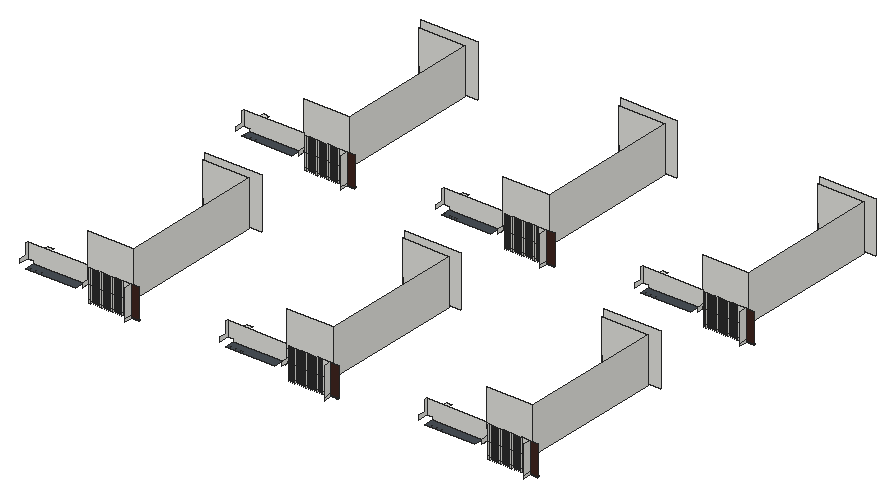
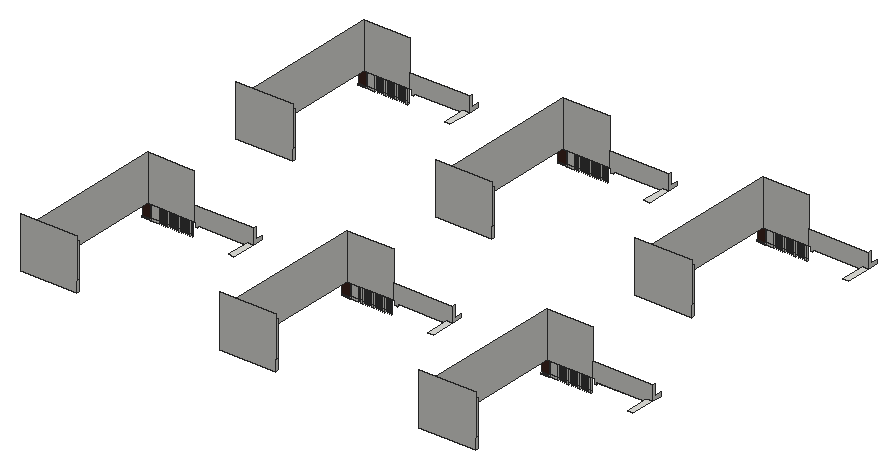
# SketchUp Ruby script. Lengths in inches.
U = 1.inch
M = Sketchup.active_model
def pt(a) = Geom::Point3d.new(a.map { |v| v * U })
def face(e, loops, mat)
  f = e.add_face(loops[0].map { |a| pt(a) })
  loops[1..].each { |l| e.add_face(l.map { |a| pt(a) }).erase! }
  f.material = f.back_material = mat if mat
  f
end
# faces: each face lists its corners as indices into pts; further lists are holes
def faces(e, pts, list, mat = nil) = list.each { |f| face(e, (f[0].is_a?(Array) ? f : [f]).map { |l| l.map { |i| pts[i] } }, mat) }
# xy, xz, yz: faces in a plane at the given z, y or x. An outline is a flat list of corners, or four numbers for a rectangle; further outlines are holes
def ring(l) = l.size == 4 ? [[l[0], l[1]], [l[2], l[1]], [l[2], l[3]], [l[0], l[3]]] : l.each_slice(2).to_a
def flat(e, list, mat, &to3) = list.each { |f| face(e, (f[0].is_a?(Array) ? f : [f]).map { |l| ring(l).map { |u, v| to3.(u, v) } }, mat) }
def xy(e, z, list, mat = nil) = flat(e, list, mat) { |x, y| [x, y, z] }
def xz(e, y, list, mat = nil) = flat(e, list, mat) { |x, z| [x, y, z] }
def yz(e, x, list, mat = nil) = flat(e, list, mat) { |y, z| [x, y, z] }
def lines(e, pts, list) = list.each { |a, b| e.add_line(pt(pts[a]), pt(pts[b])) }
# prism: a flat outline (further loops are holes) pulled along v
def prism(e, loops, v, mat = nil)
  f = face(e, loops, mat); d = Geom::Vector3d.new(v.map { |x| x * U })
  f.pushpull(f.normal.samedirection?(d) ? d.length : -d.length)
end
def box(e, o, s, mat = nil) = prism(e, [[o, [o[0] + s[0], o[1], o[2]], [o[0] + s[0], o[1] + s[1], o[2]], [o[0], o[1] + s[1], o[2]]]], [0, 0, s[2]], mat)
def at(x, y, z, deg = 0) = Geom::Transformation.translation(pt([x, y, z])) * Geom::Transformation.rotation(ORIGIN, Z_AXIS, deg.degrees)
def axes(o, x, y, z) = Geom::Transformation.new([*x, 0, *y, 0, *z, 0, *pt(o).to_a, 1])
def part(name) = M.definitions.add(name)
# library, detail: a bought-in or finely detailed component or shape, given as its bounding box
def library(name, o, s) = part(name).tap { |d| box(d.entities, o, s) }
def detail(e, o, s) = box(e.add_group.entities, o, s)
def put(e, d, t, mat = nil) = e.add_instance(d, t).tap { |i| i.material = mat if mat }
def group(e, t, mat = nil) = e.add_group.tap { |g| g.transformation = t; g.material = mat if mat }.entities
root = M.entities
M.materials.add("[0043_SaddleBrown]").color = [63, 38, 31]
M.materials.add("[Formica Blue]").color = [73, 80, 86]
xy(root,623.5625,[[517.3125,438.73,547.05,442.66],[1241.75,438.73,1271.49,442.66],[1966.1875,438.73,1995.93,442.66],[517.3125,1419.08,547.05,1423.01],[1241.75,1419.08,1271.49,1423.01],
  [1966.1875,1419.08,1995.93,1423.01]])
xy(root,626.6,[[517.3125,438.72,517.3125,442.66,547.05,442.66,547.05,438.73],[1241.75,438.72,1241.75,442.66,1271.49,442.66,1271.49,438.73],[1966.1875,438.72,1966.1875,442.66,1995.93,442.66,1995.93,438.73],[517.3125,1419.07,517.3125,1423.01,547.05,1423.01,547.05,1419.08],[1241.75,1419.07,1241.75,1423.01,1271.49,1423.01,1271.49,1419.08],
  [1966.1875,1419.07,1966.1875,1423.01,1995.93,1423.01,1995.93,1419.08]])
xy(root,669.8125,[[[158.83,412.04,338.6875,447.84],[161.79,416.2,166.6,422.7],[168.1,416.2,172.92,422.7],[174.42,416.2,179.23,422.7],[180.67,416.2,185.48,422.7],[186.92,416.2,191.73,422.7],[193.17,416.2,197.98,422.7],[199.42,416.2,204.23,422.7],[205.67,416.2,210.48,422.7],[211.92,416.2,216.73,422.7]],[[883.27,412.04,1063.125,447.84],[886.23,416.2,891.04,422.7],[892.54,416.2,897.35,422.7],[898.85,416.2,903.67,422.7],[905.1,416.2,909.92,422.7],[911.35,416.2,916.17,422.7],[917.6,416.2,922.42,422.7],[923.85,416.2,928.67,422.7],[930.1,416.2,934.92,422.7],[936.35,416.2,941.17,422.7]],[[1607.71,412.04,1787.5625,447.84],[1610.67,416.2,1615.48,422.7],[1616.98,416.2,1621.79,422.7],[1623.29,416.2,1628.1,422.7],[1629.54,416.2,1634.35,422.7],[1635.79,416.2,1640.6,422.7],[1642.04,416.2,1646.85,422.7],[1648.29,416.2,1653.1,422.7],[1654.54,416.2,1659.35,422.7],[1660.79,416.2,1665.6,422.7]],[[158.83,1392.39,338.6875,1428.19],[161.79,1396.55,166.6,1403.05],[168.1,1396.55,172.92,1403.05],[174.42,1396.55,179.23,1403.05],[180.67,1396.55,185.48,1403.05],[186.92,1396.55,191.73,1403.05],[193.17,1396.55,197.98,1403.05],[199.42,1396.55,204.23,1403.05],[205.67,1396.55,210.48,1403.05],[211.92,1396.55,216.73,1403.05]],[[883.27,1392.39,1063.125,1428.19],[886.23,1396.55,891.04,1403.05],[892.54,1396.55,897.35,1403.05],[898.85,1396.55,903.67,1403.05],[905.1,1396.55,909.92,1403.05],[911.35,1396.55,916.17,1403.05],[917.6,1396.55,922.42,1403.05],[923.85,1396.55,928.67,1403.05],[930.1,1396.55,934.92,1403.05],[936.35,1396.55,941.17,1403.05]],
  [[1607.71,1392.39,1787.5625,1428.19],[1610.67,1396.55,1615.48,1403.05],[1616.98,1396.55,1621.79,1403.05],[1623.29,1396.55,1628.1,1403.05],[1629.54,1396.55,1634.35,1403.05],[1635.79,1396.55,1640.6,1403.05],[1642.04,1396.55,1646.85,1403.05],[1648.29,1396.55,1653.1,1403.05],[1654.54,1396.55,1659.35,1403.05],[1660.79,1396.55,1665.6,1403.05]]],"[Formica Blue]")
xy(root,679.3125,[[137.5,447.84,158.83,535.375],[861.9375,447.84,883.27,535.375],[1586.375,447.84,1607.71,535.375],[137.5,1428.19,158.83,1515.73],[861.9375,1428.19,883.27,1515.73],
  [1586.375,1428.19,1607.71,1515.73]])
xz(root,438.72,[[487.0625,630.25,517.3125,679.3125],[1211.5,630.25,1241.75,679.3125],[1935.9375,630.25,1966.1875,679.3125],[487.0625,679.3125,517.3125,733.125],[1211.5,679.3125,1241.75,733.125],
  [1935.9375,679.3125,1966.1875,733.125]])
xz(root,442.66,[[517.3125,623.5625,547.05,626.6],[1241.75,623.5625,1271.49,626.6],[1966.1875,623.5625,1995.93,626.6]],"[0043_SaddleBrown]")
xz(root,447.84,[[338.6875,662.8125,338.6875,669.8125,158.83,669.8125,158.83,679.3125,137.5,679.3125,137.5,733.125,353.97,733.125,353.97,679.3125,348.1875,679.3125,348.1875,662.8125],[1063.125,662.8125,1063.125,669.8125,883.27,669.8125,883.27,679.3125,861.9375,679.3125,861.9375,733.125,1078.41,733.125,1078.41,679.3125,1072.625,679.3125,1072.625,662.8125],[1787.5625,662.8125,1787.5625,669.8125,1607.71,669.8125,1607.71,679.3125,1586.375,679.3125,1586.375,733.125,1802.84,733.125,1802.84,679.3125,1797.0625,679.3125,1797.0625,662.8125],[353.97,679.3125,521.63,845.41],[1078.41,679.3125,1246.07,845.41],
  [1802.84,679.3125,1970.51,845.41]])
xz(root,971.23,[[353.97,679.3125,521.63,845.41],[1078.41,679.3125,1246.07,845.41],[1802.84,679.3125,1970.51,845.41]])
xz(root,980.35,[[353.97,679.3125,558.625,866.5625],[1078.41,679.3125,1283.0625,866.5625],[1802.84,679.3125,2007.5,866.5625]])
xz(root,1419.07,[[487.0625,630.25,517.3125,679.3125],[1211.5,630.25,1241.75,679.3125],[1935.9375,630.25,1966.1875,679.3125],[487.0625,679.3125,517.3125,733.125],[1211.5,679.3125,1241.75,733.125],
  [1935.9375,679.3125,1966.1875,733.125]])
xz(root,1423.01,[[517.3125,623.5625,547.05,626.6],[1241.75,623.5625,1271.49,626.6],[1966.1875,623.5625,1995.93,626.6]],"[0043_SaddleBrown]")
xz(root,1428.19,[[338.6875,662.8125,338.6875,669.8125,158.83,669.8125,158.83,679.3125,137.5,679.3125,137.5,733.125,353.97,733.125,353.97,679.3125,348.1875,679.3125,348.1875,662.8125],[1063.125,662.8125,1063.125,669.8125,883.27,669.8125,883.27,679.3125,861.9375,679.3125,861.9375,733.125,1078.41,733.125,1078.41,679.3125,1072.625,679.3125,1072.625,662.8125],[1787.5625,662.8125,1787.5625,669.8125,1607.71,669.8125,1607.71,679.3125,1586.375,679.3125,1586.375,733.125,1802.84,733.125,1802.84,679.3125,1797.0625,679.3125,1797.0625,662.8125],[353.97,679.3125,521.63,845.41],[1078.41,679.3125,1246.07,845.41],
  [1802.84,679.3125,1970.51,845.41]])
xz(root,1951.58,[[353.97,679.3125,521.63,845.41],[1078.41,679.3125,1246.07,845.41],[1802.84,679.3125,1970.51,845.41]])
xz(root,1960.7,[[353.97,679.3125,558.625,866.5625],[1078.41,679.3125,1283.0625,866.5625],[1802.84,679.3125,2007.5,866.5625]])
yz(root,137.5,[[412.04,679.3125,412.04,693.65,438.72,693.65,438.72,733.125,447.84,733.125,447.84,679.3125],[1392.39,679.3125,1392.39,693.65,1419.07,693.65,1419.07,733.125,1428.19,733.125,1428.19,679.3125]])
yz(root,353.97,[[971.23,679.3125,980.35,718],[1951.58,679.3125,1960.7,718]])
yz(root,363.73,[[412.04,679.3125,437.1,693.65],[437.1,679.3125,438.72,693.65],[1392.39,679.3125,1417.45,693.65],[1417.45,679.3125,1419.07,693.65]])
yz(root,367.0625,[[437.1,620.875,438.72,630.25],[1417.45,620.875,1419.07,630.25],[437.1,630.25,438.72,679.3125],[1417.45,630.25,1419.07,679.3125],[437.1,679.3125,438.72,733.125],
  [1417.45,679.3125,1419.07,733.125]])
yz(root,375.0625,[[437.1,620.875,438.72,630.25],[1417.45,620.875,1419.07,630.25],[437.1,630.25,438.72,679.3125],[1417.45,630.25,1419.07,679.3125],[437.1,679.3125,438.72,733.125],
  [1417.45,679.3125,1419.07,733.125]])
yz(root,383.0625,[[437.1,620.875,438.72,630.25],[1417.45,620.875,1419.07,630.25],[437.1,630.25,438.72,679.3125],[1417.45,630.25,1419.07,679.3125],[437.1,679.3125,438.72,733.125],
  [1417.45,679.3125,1419.07,733.125]])
yz(root,391.0625,[[437.1,620.875,438.72,630.25],[1417.45,620.875,1419.07,630.25],[437.1,630.25,438.72,679.3125],[1417.45,630.25,1419.07,679.3125],[437.1,679.3125,438.72,733.125],
  [1417.45,679.3125,1419.07,733.125]])
yz(root,399.0625,[[437.1,620.875,438.72,630.25],[1417.45,620.875,1419.07,630.25],[437.1,630.25,438.72,679.3125],[1417.45,630.25,1419.07,679.3125],[437.1,679.3125,438.72,733.125],
  [1417.45,679.3125,1419.07,733.125]])
yz(root,407.0625,[[437.1,620.875,438.72,630.25],[1417.45,620.875,1419.07,630.25],[437.1,630.25,438.72,679.3125],[1417.45,630.25,1419.07,679.3125],[437.1,679.3125,438.72,733.125],
  [1417.45,679.3125,1419.07,733.125]])
yz(root,415.0625,[[437.1,620.875,438.72,630.25],[1417.45,620.875,1419.07,630.25],[437.1,630.25,438.72,679.3125],[1417.45,630.25,1419.07,679.3125],[437.1,679.3125,438.72,733.125],
  [1417.45,679.3125,1419.07,733.125]])
yz(root,423.0625,[[437.1,620.875,438.72,630.25],[1417.45,620.875,1419.07,630.25],[437.1,630.25,438.72,679.3125],[1417.45,630.25,1419.07,679.3125],[437.1,679.3125,438.72,733.125],
  [1417.45,679.3125,1419.07,733.125]])
yz(root,431.0625,[[437.1,620.875,438.72,630.25],[1417.45,620.875,1419.07,630.25],[437.1,630.25,438.72,679.3125],[1417.45,630.25,1419.07,679.3125],[437.1,679.3125,438.72,733.125],
  [1417.45,679.3125,1419.07,733.125]])
yz(root,439.0625,[[437.1,620.875,438.72,630.25],[1417.45,620.875,1419.07,630.25],[437.1,630.25,438.72,679.3125],[1417.45,630.25,1419.07,679.3125],[437.1,679.3125,438.72,733.125],
  [1417.45,679.3125,1419.07,733.125]])
yz(root,447.0625,[[437.1,620.875,438.72,630.25],[1417.45,620.875,1419.07,630.25],[437.1,630.25,438.72,679.3125],[1417.45,630.25,1419.07,679.3125],[437.1,679.3125,438.72,733.125],
  [1417.45,679.3125,1419.07,733.125]])
yz(root,455.0625,[[437.1,620.875,438.72,630.25],[1417.45,620.875,1419.07,630.25],[437.1,630.25,438.72,679.3125],[1417.45,630.25,1419.07,679.3125],[437.1,679.3125,438.72,733.125],
  [1417.45,679.3125,1419.07,733.125]])
yz(root,463.0625,[[437.1,620.875,438.72,630.25],[1417.45,620.875,1419.07,630.25],[437.1,630.25,438.72,679.3125],[1417.45,630.25,1419.07,679.3125],[437.1,679.3125,438.72,733.125],
  [1417.45,679.3125,1419.07,733.125]])
yz(root,471.0625,[[437.1,620.875,438.72,630.25],[1417.45,620.875,1419.07,630.25],[437.1,630.25,438.72,679.3125],[1417.45,630.25,1419.07,679.3125],[437.1,679.3125,438.72,733.125],
  [1417.45,679.3125,1419.07,733.125]])
yz(root,479.0625,[[437.1,620.875,438.72,630.25],[1417.45,620.875,1419.07,630.25],[437.1,630.25,438.72,679.3125],[1417.45,630.25,1419.07,679.3125],[437.1,679.3125,438.72,733.125],
  [1417.45,679.3125,1419.07,733.125]])
yz(root,487.0625,[[437.1,620.875,438.72,630.25],[1417.45,620.875,1419.07,630.25],[437.1,630.25,438.72,679.3125],[1417.45,630.25,1419.07,679.3125],[437.1,679.3125,438.72,733.125],
  [1417.45,679.3125,1419.07,733.125]])
yz(root,517.3125,[[412.04,620.875,438.72,620.875,438.73,623.5625,438.72,626.6,438.72,630.25,412.04,630.25],[1392.39,620.875,1419.07,620.875,1419.08,623.5625,1419.07,626.6,1419.07,630.25,1392.39,630.25],[438.73,623.5625,442.66,623.5625,442.66,626.6,438.72,626.6],[1419.08,623.5625,1423.01,623.5625,1423.01,626.6,1419.07,626.6],[412.04,630.25,438.72,733.125],
  [1392.39,630.25,1419.07,733.125]])
yz(root,521.63,[[447.84,679.3125,971.23,845.41],[1428.19,679.3125,1951.58,845.41]])
yz(root,861.9375,[[412.04,679.3125,412.04,693.65,438.72,693.65,438.72,733.125,447.84,733.125,447.84,679.3125],[1392.39,679.3125,1392.39,693.65,1419.07,693.65,1419.07,733.125,1428.19,733.125,1428.19,679.3125]])
yz(root,1078.41,[[971.23,679.3125,980.35,718],[1951.58,679.3125,1960.7,718]])
yz(root,1088.17,[[412.04,679.3125,437.1,693.65],[437.1,679.3125,438.72,693.65],[1392.39,679.3125,1417.45,693.65],[1417.45,679.3125,1419.07,693.65]])
yz(root,1091.5,[[437.1,620.875,438.72,630.25],[1417.45,620.875,1419.07,630.25],[437.1,630.25,438.72,679.3125],[1417.45,630.25,1419.07,679.3125],[437.1,679.3125,438.72,733.125],
  [1417.45,679.3125,1419.07,733.125]])
yz(root,1099.5,[[437.1,620.875,438.72,630.25],[1417.45,620.875,1419.07,630.25],[437.1,630.25,438.72,679.3125],[1417.45,630.25,1419.07,679.3125],[437.1,679.3125,438.72,733.125],
  [1417.45,679.3125,1419.07,733.125]])
yz(root,1107.5,[[437.1,620.875,438.72,630.25],[1417.45,620.875,1419.07,630.25],[437.1,630.25,438.72,679.3125],[1417.45,630.25,1419.07,679.3125],[437.1,679.3125,438.72,733.125],
  [1417.45,679.3125,1419.07,733.125]])
yz(root,1115.5,[[437.1,620.875,438.72,630.25],[1417.45,620.875,1419.07,630.25],[437.1,630.25,438.72,679.3125],[1417.45,630.25,1419.07,679.3125],[437.1,679.3125,438.72,733.125],
  [1417.45,679.3125,1419.07,733.125]])
yz(root,1123.5,[[437.1,620.875,438.72,630.25],[1417.45,620.875,1419.07,630.25],[437.1,630.25,438.72,679.3125],[1417.45,630.25,1419.07,679.3125],[437.1,679.3125,438.72,733.125],
  [1417.45,679.3125,1419.07,733.125]])
yz(root,1131.5,[[437.1,620.875,438.72,630.25],[1417.45,620.875,1419.07,630.25],[437.1,630.25,438.72,679.3125],[1417.45,630.25,1419.07,679.3125],[437.1,679.3125,438.72,733.125],
  [1417.45,679.3125,1419.07,733.125]])
yz(root,1139.5,[[437.1,620.875,438.72,630.25],[1417.45,620.875,1419.07,630.25],[437.1,630.25,438.72,679.3125],[1417.45,630.25,1419.07,679.3125],[437.1,679.3125,438.72,733.125],
  [1417.45,679.3125,1419.07,733.125]])
yz(root,1147.5,[[437.1,620.875,438.72,630.25],[1417.45,620.875,1419.07,630.25],[437.1,630.25,438.72,679.3125],[1417.45,630.25,1419.07,679.3125],[437.1,679.3125,438.72,733.125],
  [1417.45,679.3125,1419.07,733.125]])
yz(root,1155.5,[[437.1,620.875,438.72,630.25],[1417.45,620.875,1419.07,630.25],[437.1,630.25,438.72,679.3125],[1417.45,630.25,1419.07,679.3125],[437.1,679.3125,438.72,733.125],
  [1417.45,679.3125,1419.07,733.125]])
yz(root,1163.5,[[437.1,620.875,438.72,630.25],[1417.45,620.875,1419.07,630.25],[437.1,630.25,438.72,679.3125],[1417.45,630.25,1419.07,679.3125],[437.1,679.3125,438.72,733.125],
  [1417.45,679.3125,1419.07,733.125]])
yz(root,1171.5,[[437.1,620.875,438.72,630.25],[1417.45,620.875,1419.07,630.25],[437.1,630.25,438.72,679.3125],[1417.45,630.25,1419.07,679.3125],[437.1,679.3125,438.72,733.125],
  [1417.45,679.3125,1419.07,733.125]])
yz(root,1179.5,[[437.1,620.875,438.72,630.25],[1417.45,620.875,1419.07,630.25],[437.1,630.25,438.72,679.3125],[1417.45,630.25,1419.07,679.3125],[437.1,679.3125,438.72,733.125],
  [1417.45,679.3125,1419.07,733.125]])
yz(root,1187.5,[[437.1,620.875,438.72,630.25],[1417.45,620.875,1419.07,630.25],[437.1,630.25,438.72,679.3125],[1417.45,630.25,1419.07,679.3125],[437.1,679.3125,438.72,733.125],
  [1417.45,679.3125,1419.07,733.125]])
yz(root,1195.5,[[437.1,620.875,438.72,630.25],[1417.45,620.875,1419.07,630.25],[437.1,630.25,438.72,679.3125],[1417.45,630.25,1419.07,679.3125],[437.1,679.3125,438.72,733.125],
  [1417.45,679.3125,1419.07,733.125]])
yz(root,1203.5,[[437.1,620.875,438.72,630.25],[1417.45,620.875,1419.07,630.25],[437.1,630.25,438.72,679.3125],[1417.45,630.25,1419.07,679.3125],[437.1,679.3125,438.72,733.125],
  [1417.45,679.3125,1419.07,733.125]])
yz(root,1211.5,[[437.1,620.875,438.72,630.25],[1417.45,620.875,1419.07,630.25],[437.1,630.25,438.72,679.3125],[1417.45,630.25,1419.07,679.3125],[437.1,679.3125,438.72,733.125],
  [1417.45,679.3125,1419.07,733.125]])
yz(root,1241.75,[[412.04,620.875,438.72,620.875,438.73,623.5625,438.72,626.6,438.72,630.25,412.04,630.25],[1392.39,620.875,1419.07,620.875,1419.08,623.5625,1419.07,626.6,1419.07,630.25,1392.39,630.25],[438.73,623.5625,442.66,623.5625,442.66,626.6,438.72,626.6],[1419.08,623.5625,1423.01,623.5625,1423.01,626.6,1419.07,626.6],[412.04,630.25,438.72,733.125],
  [1392.39,630.25,1419.07,733.125]])
yz(root,1246.07,[[447.84,679.3125,971.23,845.41],[1428.19,679.3125,1951.58,845.41]])
yz(root,1586.375,[[412.04,679.3125,412.04,693.65,438.72,693.65,438.72,733.125,447.84,733.125,447.84,679.3125],[1392.39,679.3125,1392.39,693.65,1419.07,693.65,1419.07,733.125,1428.19,733.125,1428.19,679.3125]])
yz(root,1802.84,[[971.23,679.3125,980.35,718],[1951.58,679.3125,1960.7,718]])
yz(root,1812.6,[[412.04,679.3125,437.1,693.65],[437.1,679.3125,438.72,693.65],[1392.39,679.3125,1417.45,693.65],[1417.45,679.3125,1419.07,693.65]])
yz(root,1815.9375,[[437.1,620.875,438.72,630.25],[1417.45,620.875,1419.07,630.25],[437.1,630.25,438.72,679.3125],[1417.45,630.25,1419.07,679.3125],[437.1,679.3125,438.72,733.125],
  [1417.45,679.3125,1419.07,733.125]])
yz(root,1823.9375,[[437.1,620.875,438.72,630.25],[1417.45,620.875,1419.07,630.25],[437.1,630.25,438.72,679.3125],[1417.45,630.25,1419.07,679.3125],[437.1,679.3125,438.72,733.125],
  [1417.45,679.3125,1419.07,733.125]])
yz(root,1831.9375,[[437.1,620.875,438.72,630.25],[1417.45,620.875,1419.07,630.25],[437.1,630.25,438.72,679.3125],[1417.45,630.25,1419.07,679.3125],[437.1,679.3125,438.72,733.125],
  [1417.45,679.3125,1419.07,733.125]])
yz(root,1839.9375,[[437.1,620.875,438.72,630.25],[1417.45,620.875,1419.07,630.25],[437.1,630.25,438.72,679.3125],[1417.45,630.25,1419.07,679.3125],[437.1,679.3125,438.72,733.125],
  [1417.45,679.3125,1419.07,733.125]])
yz(root,1847.9375,[[437.1,620.875,438.72,630.25],[1417.45,620.875,1419.07,630.25],[437.1,630.25,438.72,679.3125],[1417.45,630.25,1419.07,679.3125],[437.1,679.3125,438.72,733.125],
  [1417.45,679.3125,1419.07,733.125]])
yz(root,1855.9375,[[437.1,620.875,438.72,630.25],[1417.45,620.875,1419.07,630.25],[437.1,630.25,438.72,679.3125],[1417.45,630.25,1419.07,679.3125],[437.1,679.3125,438.72,733.125],
  [1417.45,679.3125,1419.07,733.125]])
yz(root,1863.9375,[[437.1,620.875,438.72,630.25],[1417.45,620.875,1419.07,630.25],[437.1,630.25,438.72,679.3125],[1417.45,630.25,1419.07,679.3125],[437.1,679.3125,438.72,733.125],
  [1417.45,679.3125,1419.07,733.125]])
yz(root,1871.9375,[[437.1,620.875,438.72,630.25],[1417.45,620.875,1419.07,630.25],[437.1,630.25,438.72,679.3125],[1417.45,630.25,1419.07,679.3125],[437.1,679.3125,438.72,733.125],
  [1417.45,679.3125,1419.07,733.125]])
yz(root,1879.9375,[[437.1,620.875,438.72,630.25],[1417.45,620.875,1419.07,630.25],[437.1,630.25,438.72,679.3125],[1417.45,630.25,1419.07,679.3125],[437.1,679.3125,438.72,733.125],
  [1417.45,679.3125,1419.07,733.125]])
yz(root,1887.9375,[[437.1,620.875,438.72,630.25],[1417.45,620.875,1419.07,630.25],[437.1,630.25,438.72,679.3125],[1417.45,630.25,1419.07,679.3125],[437.1,679.3125,438.72,733.125],
  [1417.45,679.3125,1419.07,733.125]])
yz(root,1895.9375,[[437.1,620.875,438.72,630.25],[1417.45,620.875,1419.07,630.25],[437.1,630.25,438.72,679.3125],[1417.45,630.25,1419.07,679.3125],[437.1,679.3125,438.72,733.125],
  [1417.45,679.3125,1419.07,733.125]])
yz(root,1903.9375,[[437.1,620.875,438.72,630.25],[1417.45,620.875,1419.07,630.25],[437.1,630.25,438.72,679.3125],[1417.45,630.25,1419.07,679.3125],[437.1,679.3125,438.72,733.125],
  [1417.45,679.3125,1419.07,733.125]])
yz(root,1911.9375,[[437.1,620.875,438.72,630.25],[1417.45,620.875,1419.07,630.25],[437.1,630.25,438.72,679.3125],[1417.45,630.25,1419.07,679.3125],[437.1,679.3125,438.72,733.125],
  [1417.45,679.3125,1419.07,733.125]])
yz(root,1919.9375,[[437.1,620.875,438.72,630.25],[1417.45,620.875,1419.07,630.25],[437.1,630.25,438.72,679.3125],[1417.45,630.25,1419.07,679.3125],[437.1,679.3125,438.72,733.125],
  [1417.45,679.3125,1419.07,733.125]])
yz(root,1927.9375,[[437.1,620.875,438.72,630.25],[1417.45,620.875,1419.07,630.25],[437.1,630.25,438.72,679.3125],[1417.45,630.25,1419.07,679.3125],[437.1,679.3125,438.72,733.125],
  [1417.45,679.3125,1419.07,733.125]])
yz(root,1935.9375,[[437.1,620.875,438.72,630.25],[1417.45,620.875,1419.07,630.25],[437.1,630.25,438.72,679.3125],[1417.45,630.25,1419.07,679.3125],[437.1,679.3125,438.72,733.125],
  [1417.45,679.3125,1419.07,733.125]])
yz(root,1966.1875,[[412.04,620.875,438.72,620.875,438.73,623.5625,438.72,626.6,438.72,630.25,412.04,630.25],[1392.39,620.875,1419.07,620.875,1419.08,623.5625,1419.07,626.6,1419.07,630.25,1392.39,630.25],[438.73,623.5625,442.66,623.5625,442.66,626.6,438.72,626.6],[1419.08,623.5625,1423.01,623.5625,1423.01,626.6,1419.07,626.6],[412.04,630.25,438.72,733.125],
  [1392.39,630.25,1419.07,733.125]])
yz(root,1970.51,[[447.84,679.3125,971.23,845.41],[1428.19,679.3125,1951.58,845.41]])
p = [[517.3125,438.72,630.25],[487.0625,438.72,630.25],[487.0625,438.72,620.875],[517.3125,438.72,620.875],[517.3125,438.73,623.5625],[517.3125,438.72,626.6],
  [1241.75,438.72,630.25],[1211.5,438.72,630.25],[1211.5,438.72,620.875],[1241.75,438.72,620.875],[1241.75,438.73,623.5625],[1241.75,438.72,626.6],
  [1966.1875,438.72,630.25],[1935.9375,438.72,630.25],[1935.9375,438.72,620.875],[1966.1875,438.72,620.875],[1966.1875,438.73,623.5625],[1966.1875,438.72,626.6],
  [517.3125,1419.07,630.25],[487.0625,1419.07,630.25],[487.0625,1419.07,620.875],[517.3125,1419.07,620.875],[517.3125,1419.08,623.5625],[517.3125,1419.07,626.6],
  [1241.75,1419.07,630.25],[1211.5,1419.07,630.25],[1211.5,1419.07,620.875],[1241.75,1419.07,620.875],[1241.75,1419.08,623.5625],[1241.75,1419.07,626.6],
  [1966.1875,1419.07,630.25],[1935.9375,1419.07,630.25],[1935.9375,1419.07,620.875],[1966.1875,1419.07,620.875],[1966.1875,1419.08,623.5625],[1966.1875,1419.07,626.6],
  [547.05,438.73,626.6],[547.05,438.72,733.125],[517.3125,438.72,733.125],[517.3125,438.72,679.3125],[1271.49,438.73,626.6],[1271.49,438.72,733.125],
  [1241.75,438.72,733.125],[1241.75,438.72,679.3125],[1995.93,438.73,626.6],[1995.93,438.72,733.125],[1966.1875,438.72,733.125],[1966.1875,438.72,679.3125],
  [547.05,1419.08,626.6],[547.05,1419.07,733.125],[517.3125,1419.07,733.125],[517.3125,1419.07,679.3125],[1271.49,1419.08,626.6],[1271.49,1419.07,733.125],
  [1241.75,1419.07,733.125],[1241.75,1419.07,679.3125],[1995.93,1419.08,626.6],[1995.93,1419.07,733.125],[1966.1875,1419.07,733.125],[1966.1875,1419.07,679.3125],
  [883.27,438.72,679.3125],[883.27,447.84,679.3125],[1607.71,438.72,679.3125],[1607.71,447.84,679.3125],[158.83,438.72,679.3125],[158.83,447.84,679.3125],
  [883.27,1419.07,679.3125],[883.27,1428.19,679.3125],[1607.71,1419.07,679.3125],[1607.71,1428.19,679.3125],[158.83,1419.07,679.3125],[158.83,1428.19,679.3125]]
faces(root,p,[[0,1,2,3,4,5],[6,7,8,9,10,11],[12,13,14,15,16,17],[18,19,20,21,22,23],[24,25,26,27,28,29],[30,31,32,33,34,35]])
faces(root,p,[[36,37,38,39,0,5],[40,41,42,43,6,11],[44,45,46,47,12,17],[48,49,50,51,18,23],[52,53,54,55,24,29],[56,57,58,59,30,35]],"[0043_SaddleBrown]")
lines(root,p,[[60,61],[62,63],[64,65],[66,67],[68,69],[70,71]])
